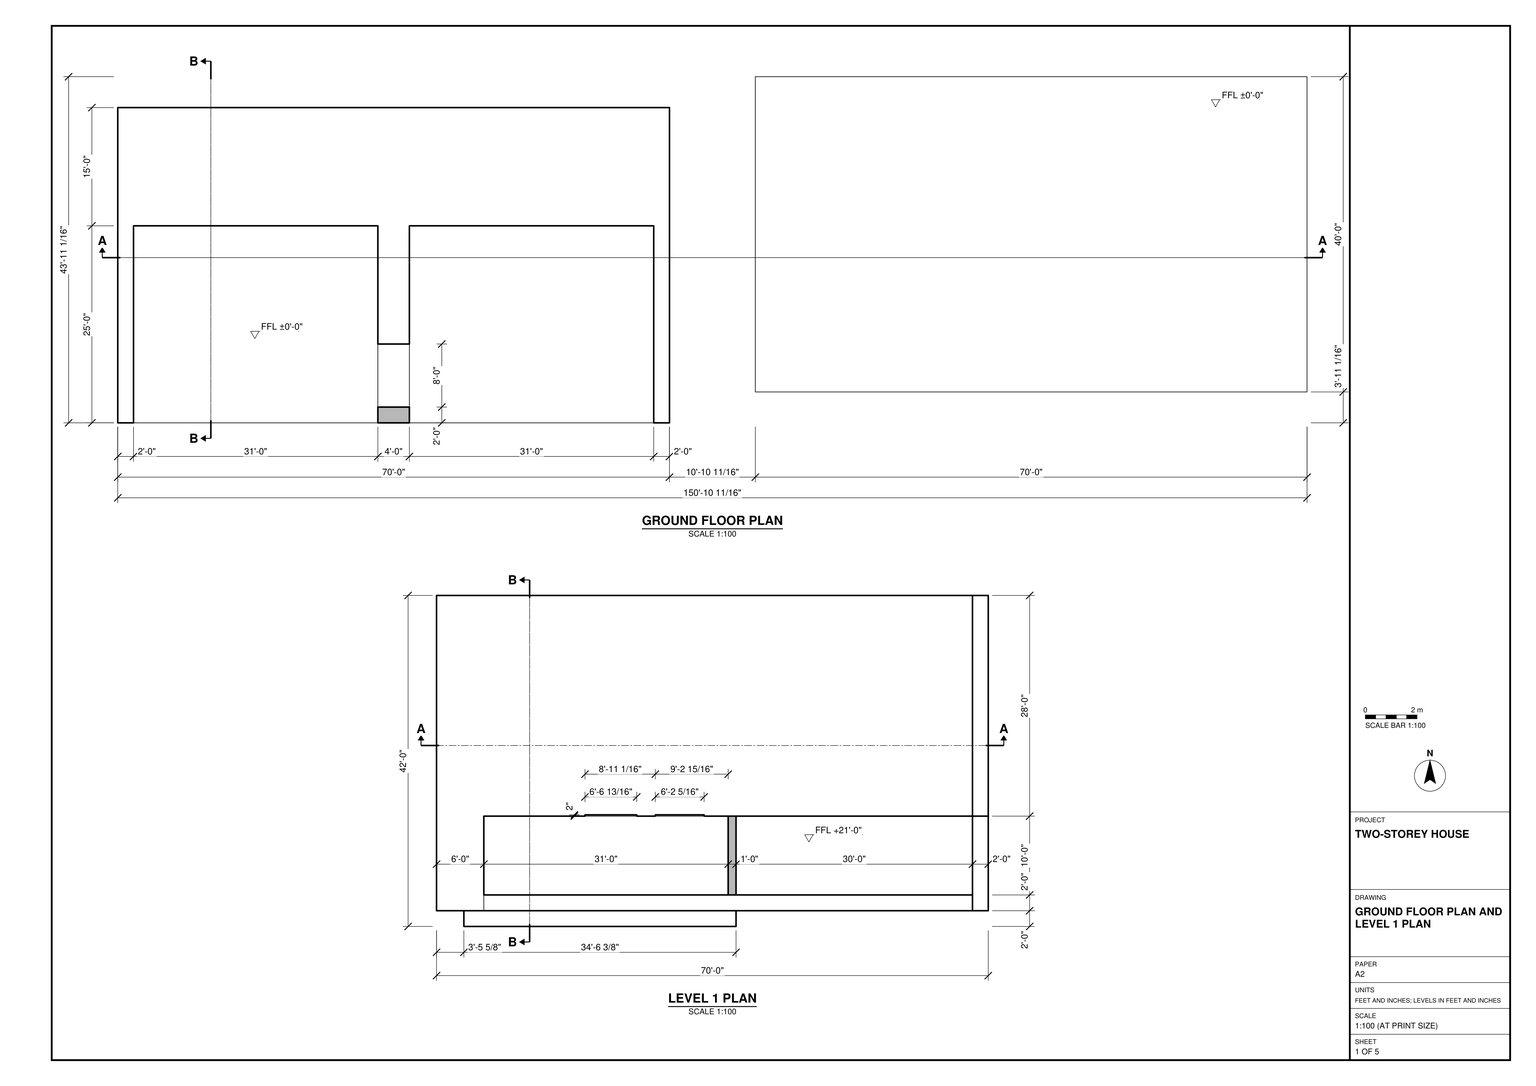
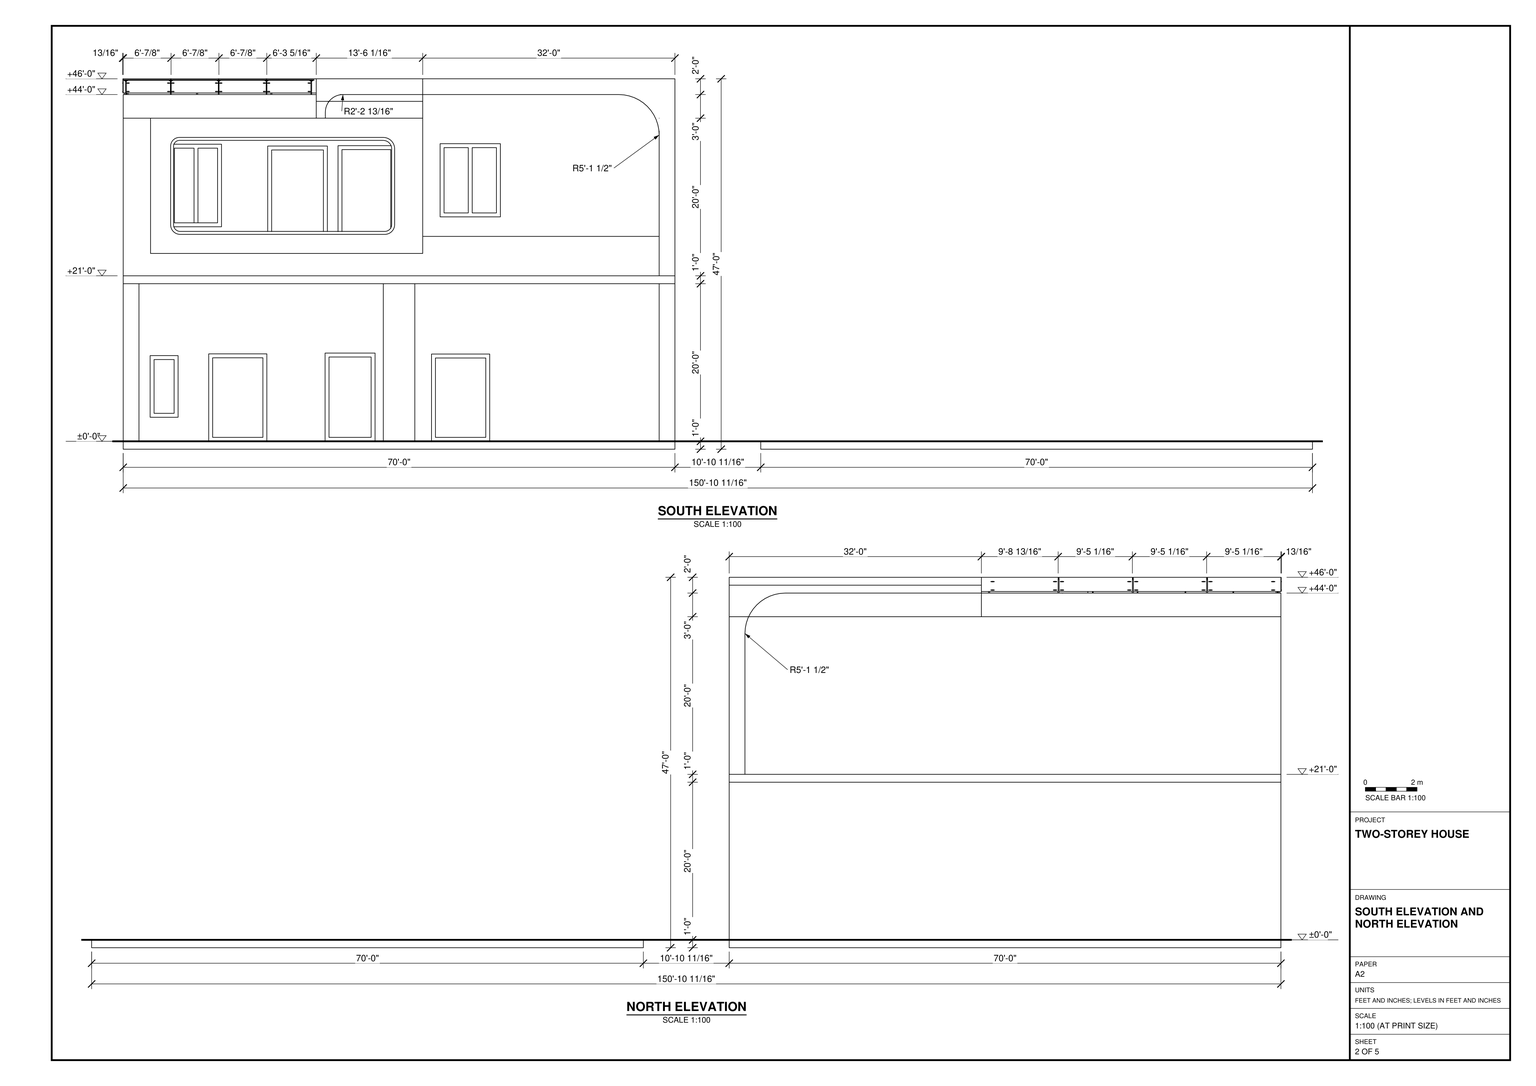
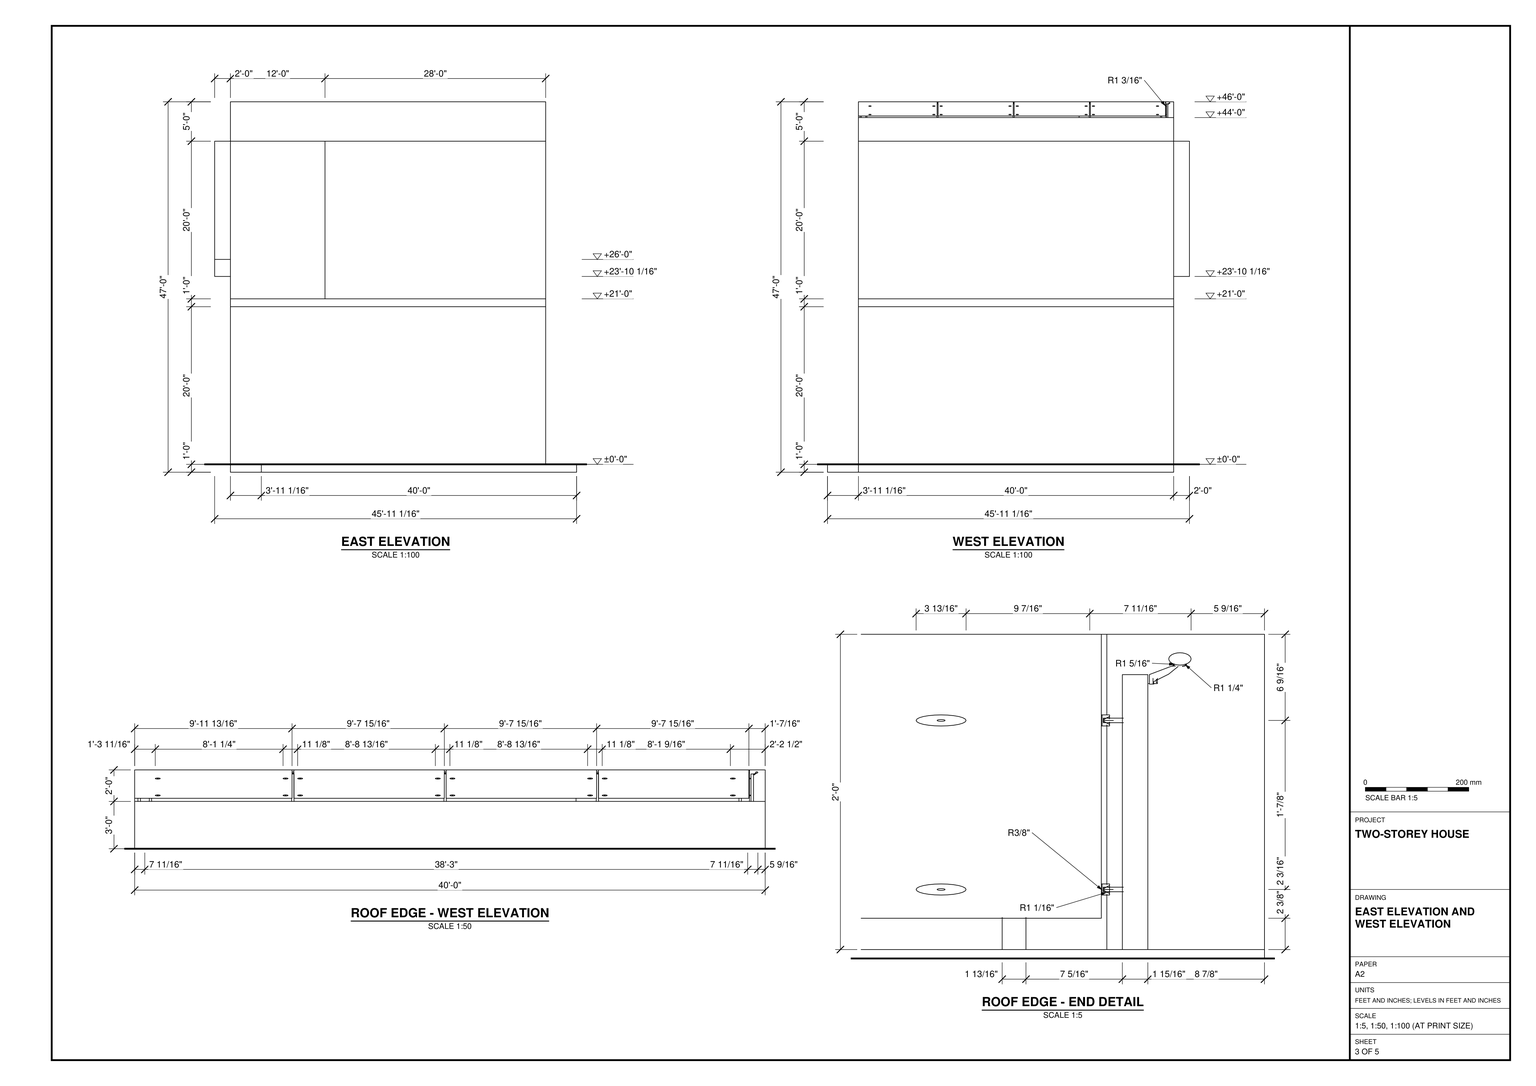
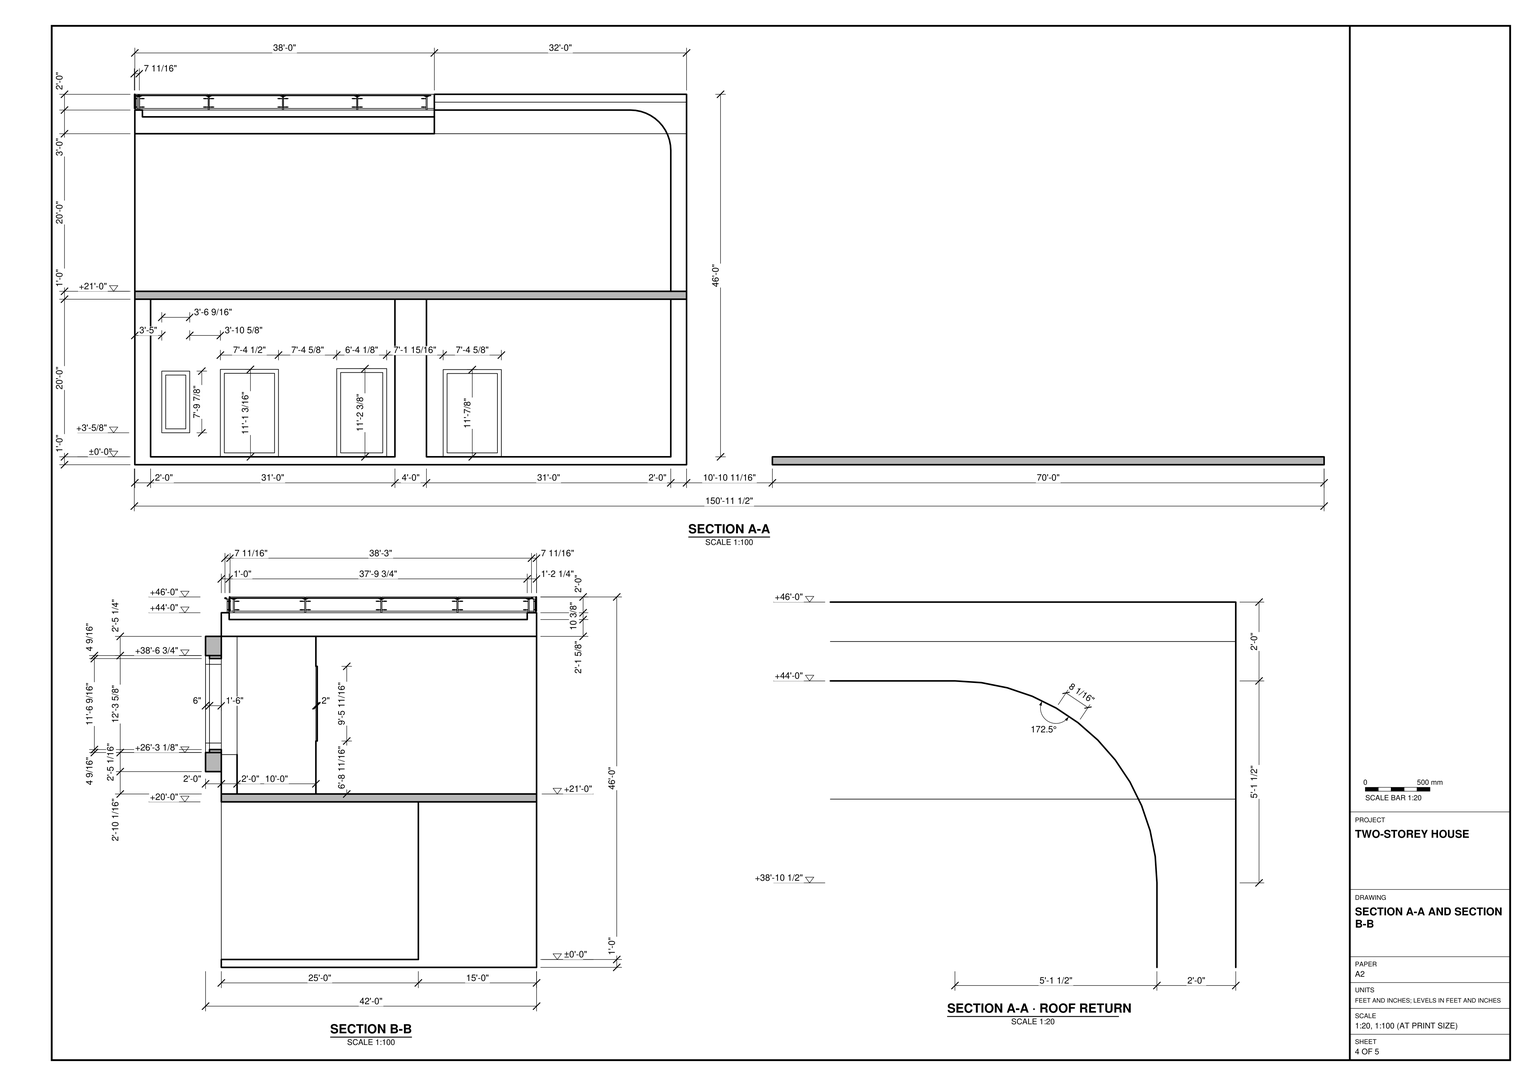
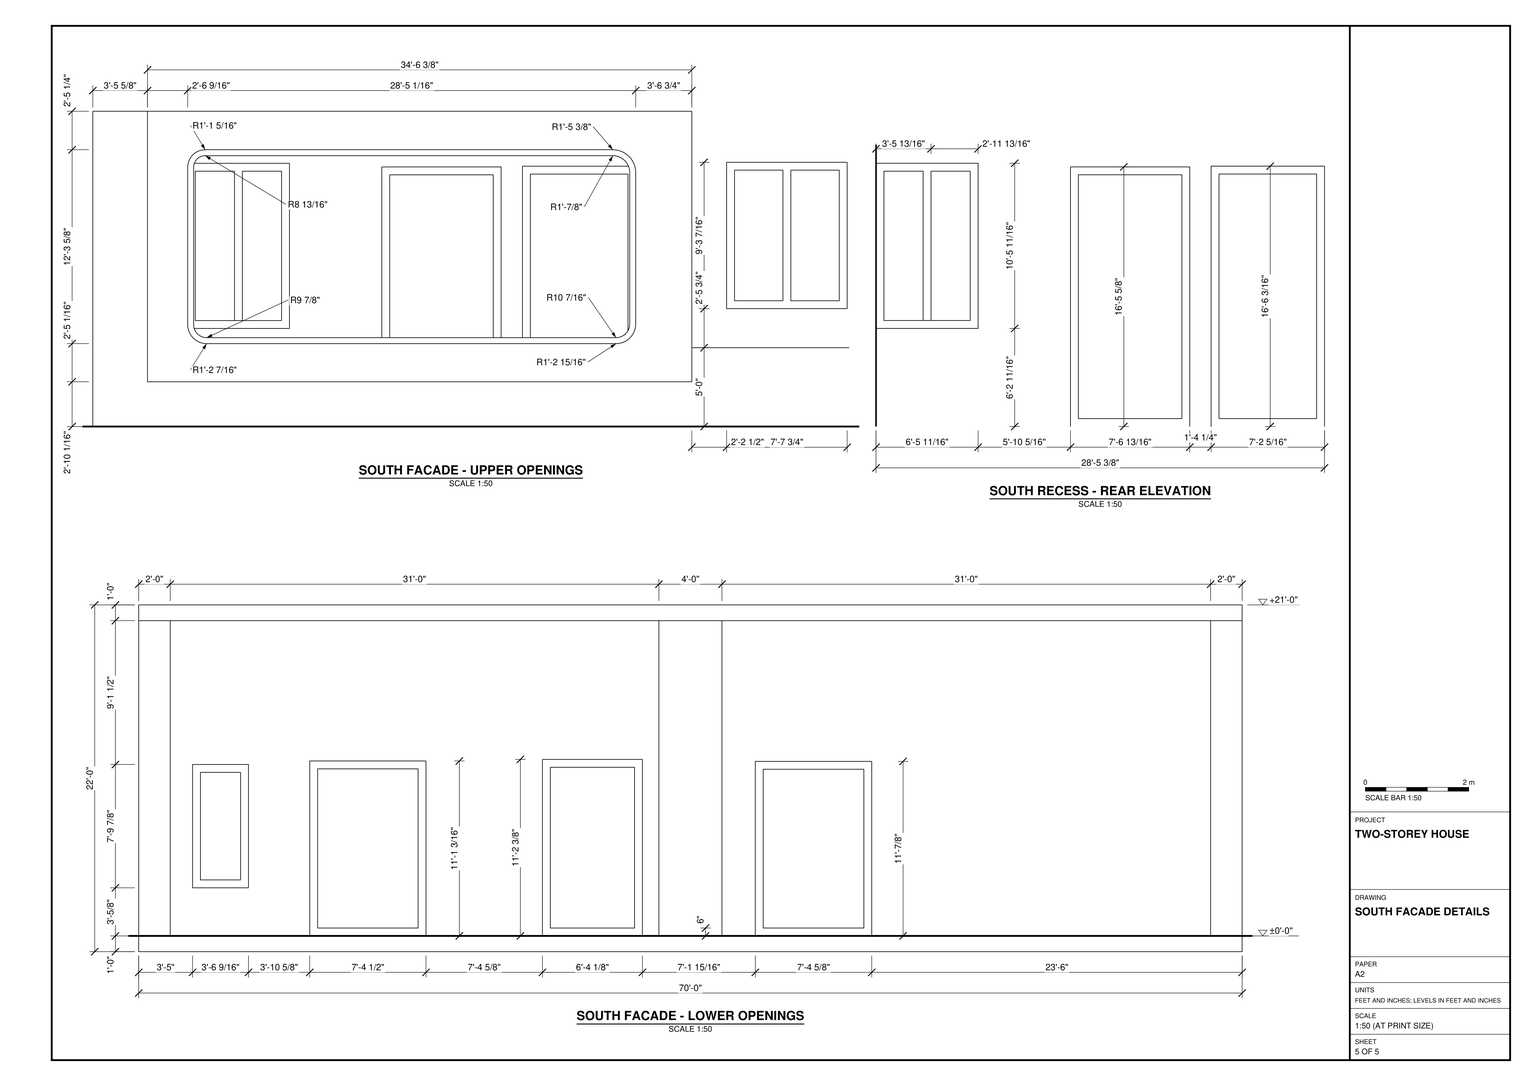
Build the two-storey house and the separate rectangular ground slab shown in task_files/diagram_01.pdf. Work in feet and inches. The complete model, including the offset slab, measures 150'-11 1/2" along X, 45'-11 1/16" along Y and 47'-0" along Z. Set the ground finished floor at ±0'-0" and the upper finished floor at +21'-0".

Use the ground floor plan to place the slab east of the house, with the gap and the northward offset shown. Build the walls, supports, floor slabs and flat roof to the thicknesses drawn. Form the two recessed bays on the south side and place the framed door and window openings on the walls behind the supports. On the upper storey, model the projecting surround with its rounded rectangular opening, keeping it distinct from the openings behind it. Form the curved return where the roof meets the right side of the south elevation. Use the roof-edge detail to model the glass guard panels, their point fixings and the handrail above the solid roof-edge band.

Keep walls, slabs and roof elements in separate groups or components. Keep any furniture or joinery piece separate and use components for repeated parts such as guard fittings. Any decor or loose items shown may be suitable library components. Save one SketchUp model as output_files/two_storey_house_with_a_glazed_roof_edge_guard.skp.

# SketchUp Ruby script. Lengths in inches.
U = 1.inch
M = Sketchup.active_model
def pt(a) = Geom::Point3d.new(a.map { |v| v * U })
def face(e, loops, mat)
  f = e.add_face(loops[0].map { |a| pt(a) })
  loops[1..].each { |l| e.add_face(l.map { |a| pt(a) }).erase! }
  f.material = f.back_material = mat if mat
  f
end
# faces: each face lists its corners as indices into pts; further lists are holes
def faces(e, pts, list, mat = nil) = list.each { |f| face(e, (f[0].is_a?(Array) ? f : [f]).map { |l| l.map { |i| pts[i] } }, mat) }
# xy, xz, yz: faces in a plane at the given z, y or x. An outline is a flat list of corners, or four numbers for a rectangle; further outlines are holes
def ring(l) = l.size == 4 ? [[l[0], l[1]], [l[2], l[1]], [l[2], l[3]], [l[0], l[3]]] : l.each_slice(2).to_a
def flat(e, list, mat, &to3) = list.each { |f| face(e, (f[0].is_a?(Array) ? f : [f]).map { |l| ring(l).map { |u, v| to3.(u, v) } }, mat) }
def xy(e, z, list, mat = nil) = flat(e, list, mat) { |x, y| [x, y, z] }
def xz(e, y, list, mat = nil) = flat(e, list, mat) { |x, z| [x, y, z] }
def yz(e, x, list, mat = nil) = flat(e, list, mat) { |y, z| [x, y, z] }
def lines(e, pts, list) = list.each { |a, b| e.add_line(pt(pts[a]), pt(pts[b])) }
# prism: a flat outline (further loops are holes) pulled along v
def prism(e, loops, v, mat = nil)
  f = face(e, loops, mat); d = Geom::Vector3d.new(v.map { |x| x * U })
  f.pushpull(f.normal.samedirection?(d) ? d.length : -d.length)
end
def box(e, o, s, mat = nil) = prism(e, [[o, [o[0] + s[0], o[1], o[2]], [o[0] + s[0], o[1] + s[1], o[2]], [o[0], o[1] + s[1], o[2]]]], [0, 0, s[2]], mat)
def at(x, y, z, deg = 0) = Geom::Transformation.translation(pt([x, y, z])) * Geom::Transformation.rotation(ORIGIN, Z_AXIS, deg.degrees)
def axes(o, x, y, z) = Geom::Transformation.new([*x, 0, *y, 0, *z, 0, *pt(o).to_a, 1])
def part(name) = M.definitions.add(name)
# library, detail: a bought-in or finely detailed component or shape, given as its bounding box
def library(name, o, s) = part(name).tap { |d| box(d.entities, o, s) }
def detail(e, o, s) = box(e.add_group.entities, o, s)
def put(e, d, t, mat = nil) = e.add_instance(d, t).tap { |i| i.material = mat if mat }
def group(e, t, mat = nil) = e.add_group.tap { |g| g.transformation = t; g.material = mat if mat }.entities
root = M.entities
M.materials.add("Translucent_Glass_Blue").color = [72, 237, 225]
M.materials["Translucent_Glass_Blue"].alpha = 0.08
M.materials.add("[0033_NavajoWhite]").color = [255, 222, 173]
M.materials.add("[0050_LemonChiffon]").color = [209, 205, 168]
M.materials.add("[Cladding Siding Tan]").color = [141, 143, 162]
M.materials.add("[Color I01]").color = [147, 170, 198]
M.materials.add("[Color I01]1").color = [97, 111, 135]
M.materials.add("[Color I08]").color = [0, 0, 102]
M.materials.add("[Color J01]").color = [174, 200, 234]
M.materials.add("[Color_002]").color = [198, 198, 198]
M.materials.add("[Color_007]").color = [89, 89, 89]
M.materials.add("[Wood_Cherry_Original]").color = [181, 109, 60]
c1 = library("componance C-15 handrail bracket",[0,0,0],[4.12,3.04,2.87])
c2 = library("C-13 Full Assembly",[0,0,0],[6.77,4.22,1.58])
c3 = part("C-13 Gasket")
prism(c3.entities,[[[0.79,0.0625,1.57],[0.99,0.0625,1.55],[1.18,0.0625,1.47],[1.34,0.0625,1.34],[1.47,0.0625,1.18],[1.55,0.0625,0.99],[1.57,0.0625,0.79],[1.55,0.0625,0.58],[1.47,0.0625,0.39],[1.34,0.0625,0.23],[1.18,0.0625,0.11],[0.99,0.0625,0.03],[0.79,0.0625,0],[0.58,0.0625,0.03],[0.39,0.0625,0.11],[0.23,0.0625,0.23],[0.11,0.0625,0.39],[0.03,0.0625,0.58],[0,0.0625,0.79],[0.03,0.0625,0.99],[0.11,0.0625,1.18],[0.23,0.0625,1.34],[0.39,0.0625,1.47],[0.58,0.0625,1.55]],[[0.91,0.0625,0.75],[0.91,0.0625,0.79],[0.91,0.0625,0.82],[0.9,0.0625,0.85],[0.875,0.0625,0.875],[0.85,0.0625,0.9],[0.82,0.0625,0.91],[0.79,0.0625,0.91],[0.75,0.0625,0.91],[0.72,0.0625,0.9],[0.7,0.0625,0.875],[0.68,0.0625,0.85],[0.67,0.0625,0.82],[0.66,0.0625,0.79],[0.67,0.0625,0.75],[0.68,0.0625,0.72],[0.7,0.0625,0.7],[0.72,0.0625,0.68],[0.75,0.0625,0.67],[0.79,0.0625,0.66],[0.82,0.0625,0.67],[0.85,0.0625,0.68],[0.875,0.0625,0.7],[0.9,0.0625,0.72]]],[0,-0.0625,0],"[Color_007]")
c4 = library("C-13 C",[0,0,0],[3.01,3.25,1.57])
c5 = library("componance half c-13",[0,0,0],[3.01,4.22,1.57])
c6 = part("C-13 Button")
prism(c6.entities,[[[0.79,0.34,1.57],[0.99,0.34,1.55],[1.18,0.34,1.47],[1.34,0.34,1.34],[1.47,0.34,1.18],[1.55,0.34,0.99],[1.57,0.34,0.79],[1.55,0.34,0.58],[1.47,0.34,0.39],[1.34,0.34,0.23],[1.18,0.34,0.11],[0.99,0.34,0.03],[0.79,0.34,0],[0.58,0.34,0.03],[0.39,0.34,0.11],[0.23,0.34,0.23],[0.11,0.34,0.39],[0.03,0.34,0.58],[0,0.34,0.79],[0.03,0.34,0.99],[0.11,0.34,1.18],[0.23,0.34,1.34],[0.39,0.34,1.47],[0.58,0.34,1.55]],[[0.91,0.34,0.79],[0.91,0.34,0.82],[0.9,0.34,0.85],[0.875,0.34,0.875],[0.85,0.34,0.9],[0.82,0.34,0.91],[0.79,0.34,0.91],[0.75,0.34,0.91],[0.72,0.34,0.9],[0.7,0.34,0.875],[0.68,0.34,0.85],[0.67,0.34,0.82],[0.66,0.34,0.79],[0.67,0.34,0.75],[0.68,0.34,0.72],[0.7,0.34,0.7],[0.72,0.34,0.68],[0.75,0.34,0.67],[0.79,0.34,0.66],[0.82,0.34,0.67],[0.85,0.34,0.68],[0.875,0.34,0.7],[0.9,0.34,0.72],[0.91,0.34,0.75]]],[0,-0.34,0],"[Color_002]")
c7 = part("Group\#3")
box(c7.entities,[65.66,0.29,4.71],[64.85,0.35,42.74],"Translucent_Glass_Blue")
prism(c7.entities,[[[261.82,4.8125,42.85],[261.82,4.97,42.82],[261.82,5.13,42.85],[261.82,5.28,42.94],[261.82,5.41,43.09],[261.82,5.51,43.28],[261.82,5.57,43.51],[261.82,5.59,43.75],[261.82,5.57,43.99],[261.82,5.51,44.21],[261.82,5.41,44.4],[261.82,5.28,44.55],[261.82,5.13,44.64],[261.82,4.97,44.67],[261.82,4.8125,44.64],[261.82,4.67,44.55],[261.82,4.54,44.4],[261.82,4.44,44.21],[261.82,4.38,43.99],[261.82,4.36,43.75],[261.82,4.38,43.51],[261.82,4.44,43.28],[261.82,4.54,43.09],[261.82,4.67,42.94]]],[-261.82,0,0],"[Wood_Cherry_Original]")
box(c7.entities,[131.31,0.29,4.71],[64.86,0.35,42.74],"Translucent_Glass_Blue")
box(c7.entities,[0,0.29,4.71],[64.86,0.35,42.74],"Translucent_Glass_Blue")
box(c7.entities,[196.97,0.29,4.71],[67.85,0.35,42.74],"Translucent_Glass_Blue")
xy(c7.entities,41.38,[[3.25,1.8,4.27,3.2],[64.8,1.8,65.83,3.2],[130.46,1.8,131.48,3.2],[196.11,1.8,197.14,3.2],[257.49,1.8,258.52,3.2]])
xz(c7.entities,1.8,[[3.25,0,4.27,41.38],[64.8,0,65.83,41.38],[130.46,0,131.48,41.38],[196.11,0,197.14,41.38],[257.49,0,258.52,41.38]])
xz(c7.entities,3.2,[[3.25,0,4.27,41.38],[64.8,0,65.83,41.38],[130.46,0,131.48,41.38],[196.11,0,197.14,41.38],[257.49,0,258.52,41.38]])
yz(c7.entities,3.25,[[1.8,0,3.2,41.38]])
yz(c7.entities,4.27,[[1.8,0,3.2,41.38]])
yz(c7.entities,64.8,[[1.8,0,3.2,35.02],[1.8,35.02,3.2,41.38]])
yz(c7.entities,65.83,[[1.8,0,3.2,35.02],[1.8,35.02,3.2,41.38]])
yz(c7.entities,130.46,[[1.8,0,3.2,35.02],[1.8,35.02,3.2,41.38]])
yz(c7.entities,131.48,[[1.8,0,3.2,41.38]])
yz(c7.entities,196.11,[[1.8,0,3.2,35.02],[1.8,35.02,3.2,41.38]])
yz(c7.entities,197.14,[[1.8,0,3.2,35.02],[1.8,35.02,3.2,41.38]])
yz(c7.entities,257.49,[[1.8,0,3.2,41.38]])
yz(c7.entities,258.52,[[1.8,0,3.2,41.38]])
p = [[196.85,0.29,4.71],[196.85,0.64,4.71],[65.54,0.29,4.71],[65.54,0.64,4.71]]
lines(c7.entities,p,[[0,1],[2,3]])
put(c7.entities,c1,axes([260.83,5.34,39.95],[-1.36782,0,0],[0,-0.7031,0],[0,0,1.06018]))
put(c7.entities,c2,axes([60.68,0,33.65],[1.36782,0,0],[0,0.7031,0],[0,0,1.06018]))
put(c7.entities,c2,axes([192,0,33.65],[1.36782,0,0],[0,0.7031,0],[0,0,1.06018]))
put(c7.entities,c1,axes([133.79,5.34,39.95],[-1.36782,0,0],[0,-0.7031,0],[0,0,1.06018]))
put(c7.entities,c1,axes([6.58,5.34,39.95],[-1.36782,0,0],[0,-0.7031,0],[0,0,1.06018]))
put(c7.entities,c3,axes([253.78,0.24,33.66],[1.36782,0,0],[0,0.7031,0],[0,0,1.06018]))
put(c7.entities,c2,axes([60.68,0,8.21],[1.36782,0,0],[0,0.7031,0],[0,0,1.06018]))
put(c7.entities,c4,axes([253.375,0.68,8.21],[1.36782,0,0],[0,0.7031,0],[0,0,1.06018]))
put(c7.entities,c5,axes([4.27,0,33.65],[1.36782,0,0],[0,0.7031,0],[0,0,1.06018]))
put(c7.entities,c6,axes([253.78,0,33.66],[1.36782,0,0],[0,0.7031,0],[0,0,1.06018]))
put(c7.entities,c3,axes([253.78,0.64,33.66],[1.36782,0,0],[0,0.7031,0],[0,0,1.06018]))
put(c7.entities,c2,axes([192,0,8.21],[1.36782,0,0],[0,0.7031,0],[0,0,1.06018]))
put(c7.entities,c2,axes([126.34,0,33.65],[1.36782,0,0],[0,0.7031,0],[0,0,1.06018]))
put(c7.entities,c2,axes([126.34,0,8.21],[1.36782,0,0],[0,0.7031,0],[0,0,1.06018]))
put(c7.entities,c5,axes([4.27,0,8.21],[1.36782,0,0],[0,0.7031,0],[0,0,1.06018]))
put(c7.entities,c6,axes([253.78,0,8.21],[1.36782,0,0],[0,0.7031,0],[0,0,1.06018]))
put(c7.entities,c3,axes([253.78,0.24,8.21],[1.36782,0,0],[0,0.7031,0],[0,0,1.06018]))
put(c7.entities,c4,axes([253.375,0.68,33.66],[1.36782,0,0],[0,0.7031,0],[0,0,1.06018]))
put(c7.entities,c1,axes([199.45,5.34,39.95],[-1.36782,0,0],[0,-0.7031,0],[0,0,1.06018]))
put(c7.entities,c3,axes([253.78,0.64,8.21],[1.36782,0,0],[0,0.7031,0],[0,0,1.06018]))
put(c7.entities,c1,axes([68.14,5.34,39.95],[-1.36782,0,0],[0,-0.7031,0],[0,0,1.06018]))
xy(root,0,[[0.82,24,840.82,504]])
xy(root,12,[[396.82,24,444.82,48],[396.82,48,444.82,144]])
xy(root,12,[[24.82,24,396.82,324],[444.82,24,816.82,324]],"[0033_NavajoWhite]")
xy(root,252,[[0.82,24,0.82,504,840.82,504,840.82,24,816.82,24,816.82,324,24.82,324,24.82,24],[396.82,24,444.82,48],[396.82,144,444.82,324],[396.82,144,444.82,324]])
xy(root,252,[[24.82,24,24.82,324,396.82,324,396.82,144,444.82,144,444.82,324,816.82,324,816.82,24,444.82,24,444.82,48,396.82,48,396.82,24]],"[0033_NavajoWhite]")
xy(root,264,[[0.82,24,0.82,504,840.82,504,840.82,168,72.82,168,72.82,24],[72.82,24,816.82,48],[816.82,24,840.82,168],[456.82,48,816.82,168]])
xy(root,264,[[72.82,48,444.82,168]],"[0033_NavajoWhite]")
xy(root,264.01,[[816.82,24,840.82,168],[816.82,168,840.82,504]])
xy(root,270,[[226.82,168,305.63,170],[333.89,168,408.2,170]])
xy(root,298.0625,[[42.44,0,456.82,24]])
xy(root,324,[[456.82,24,816.82,48]],"[Color J01]")
xy(root,327.11,[[87.47,6,399.125,24]])
xy(root,327.11,[[87.47,0,399.125,6]],"[Color I01]")
xy(root,331.65,[[87.47,6,399.125,24]],"[0033_NavajoWhite]")
xy(root,344.67,[[114.66,168,144.5,170]])
xy(root,359.74,[[489.31,168,526.18,170],[532.18,168,569.06,170]])
xy(root,455.625,[[226.82,168,305.63,170]])
xy(root,456.1875,[[333.89,168,408.2,170]])
xy(root,458.37,[[114.66,168,144.5,170]])
xy(root,459.18,[[489.31,168,526.18,170],[532.18,168,569.06,170]])
xy(root,470.19,[[86.36,6,396.6875,24]],"[0033_NavajoWhite]")
xy(root,474.73,[[86.36,6,396.6875,24]])
xy(root,474.73,[[86.36,0,396.6875,6]],"[Color I01]")
xy(root,504,[[42.44,0,72.82,24],[72.82,0,444.82,24],[444.82,0,456.82,24],[444.82,24,456.82,48],[444.82,48,456.82,168]])
xy(root,504,[[0.82,24,0.82,504,456.82,504,456.82,168,72.82,168,72.82,24],[72.82,24,444.82,168]],"[0033_NavajoWhite]")
xy(root,529.625,[[314.21,24,456.82,24,456.82,489.75,12.38,489.75,12.38,36,314.21,36],[294.75,24,313.1,36],[313.1,24,314.21,36]])
xy(root,540.01,[[0.82,24,294.75,24,294.75,36,12.38,36,12.38,489.75,456.82,489.75,456.82,504,0.82,504],[335.39,24,456.82,36]])
xy(root,540.01,[[456.82,24,755.31,504]],"[Color J01]")
xy(root,564.01,[[294.75,24,456.82,36],[456.82,24,840.82,504]])
xz(root,0,[[[42.44,298.0625,456.82,504],[87.47,327.11,85.59,327.23,83.73,327.6,81.94,328.21,80.25,329.05,78.68,330.09,77.26,331.34,76.01,332.76,74.96,334.33,74.125,336.03,73.52,337.82,73.15,339.67,73.03,341.55,73.03,461.4,73.14,463.14,73.48,464.85,74.04,466.5,74.8125,468.07,75.78,469.52,76.93,470.83,78.24,471.98,79.69,472.95,81.26,473.72,82.91,474.28,84.62,474.62,86.36,474.73,396.6875,474.73,398.96,474.59,401.19,474.14,403.35,473.41,405.39,472.4,407.28,471.14,408.99,469.64,410.49,467.93,411.76,466.03,412.76,463.99,413.5,461.84,413.94,459.6,414.09,457.33,414.09,342.07,413.96,340.12,413.58,338.2,412.95,336.35,412.08,334.59,411,332.96,409.71,331.49,408.23,330.2,406.61,329.11,404.85,328.25,403,327.62,401.08,327.24,399.125,327.11]]],"[Color I01]")
xz(root,6,[[[87.47,327.11,399.125,327.11,401.08,327.24,403,327.62,404.85,328.25,406.61,329.11,408.23,330.2,409.71,331.49,411,332.96,412.08,334.59,412.95,336.35,413.58,338.2,413.96,340.12,414.09,342.07,414.09,457.33,413.94,459.6,413.5,461.84,412.76,463.99,411.76,466.03,410.49,467.93,408.99,469.64,407.28,471.14,405.39,472.4,403.35,473.41,401.19,474.14,398.96,474.59,396.6875,474.73,86.36,474.73,84.62,474.62,82.91,474.28,81.26,473.72,79.69,472.95,78.24,471.98,76.93,470.83,75.78,469.52,74.8125,468.07,74.04,466.5,73.48,464.85,73.14,463.14,73.03,461.4,73.03,341.55,73.15,339.67,73.52,337.82,74.125,336.03,74.96,334.33,76.01,332.76,77.26,331.34,78.68,330.09,80.25,329.05,81.94,328.21,83.73,327.6,85.59,327.23],[87.47,331.65,86.18,331.73,84.91,331.99,83.68,332.4,82.52,332.98,81.44,333.7,80.47,334.55,79.61,335.53,78.89,336.6,78.32,337.76,77.9,338.99,77.65,340.26,77.57,341.55,77.57,461.4,77.64,462.55,77.87,463.68,78.24,464.77,78.75,465.8,79.38,466.75,80.14,467.62,81.01,468.38,81.96,469.02,83,469.52,84.09,469.89,85.21,470.12,86.36,470.19,396.6875,470.19,398.37,470.08,400.02,469.76,401.61,469.22,403.12,468.47,404.52,467.54,405.78,466.43,406.89,465.16,407.83,463.76,408.57,462.26,409.11,460.66,409.4375,459.01,409.55,457.33,409.55,342.07,409.46,340.71,409.19,339.375,408.76,338.09,408.15,336.86,407.39,335.73,406.5,334.7,405.47,333.8,404.34,333.05,403.11,332.44,401.82,332.01,400.49,331.74,399.125,331.65]]],"[0050_LemonChiffon]")
xz(root,24,[[0.82,252,840.82,264],[816.82,264,840.82,264.01],[[42.44,298.0625,456.82,504],[87.47,327.11,399.125,327.11,401.08,327.24,403,327.62,404.85,328.25,406.61,329.11,408.23,330.2,409.71,331.49,411,332.96,412.08,334.59,412.95,336.35,413.58,338.2,413.96,340.12,414.09,342.07,414.09,457.33,413.94,459.6,413.5,461.84,412.76,463.99,411.76,466.03,410.49,467.93,408.99,469.64,407.28,471.14,405.39,472.4,403.35,473.41,401.19,474.14,398.96,474.59,396.6875,474.73,86.36,474.73,84.62,474.62,82.91,474.28,81.26,473.72,79.69,472.95,78.24,471.98,76.93,470.83,75.78,469.52,74.8125,468.07,74.04,466.5,73.48,464.85,73.14,463.14,73.03,461.4,73.03,341.55,73.15,339.67,73.52,337.82,74.125,336.03,74.96,334.33,76.01,332.76,77.26,331.34,78.68,330.09,80.25,329.05,81.94,328.21,83.73,327.6,85.59,327.23]],[[87.47,327.11,85.59,327.23,83.73,327.6,81.94,328.21,80.25,329.05,78.68,330.09,77.26,331.34,76.01,332.76,74.96,334.33,74.125,336.03,73.52,337.82,73.15,339.67,73.03,341.55,73.03,461.4,73.14,463.14,73.48,464.85,74.04,466.5,74.8125,468.07,75.78,469.52,76.93,470.83,78.24,471.98,79.69,472.95,81.26,473.72,82.91,474.28,84.62,474.62,86.36,474.73,396.6875,474.73,398.96,474.59,401.19,474.14,403.35,473.41,405.39,472.4,407.28,471.14,408.99,469.64,410.49,467.93,411.76,466.03,412.76,463.99,413.5,461.84,413.94,459.6,414.09,457.33,414.09,342.07,413.96,340.12,413.58,338.2,412.95,336.35,412.08,334.59,411,332.96,409.71,331.49,408.23,330.2,406.61,329.11,404.85,328.25,403,327.62,401.08,327.24,399.125,327.11],[87.47,331.65,399.125,331.65,400.49,331.74,401.82,332.01,403.11,332.44,404.34,333.05,405.47,333.8,406.5,334.7,407.39,335.73,408.15,336.86,408.76,338.09,409.19,339.375,409.46,340.71,409.55,342.07,409.55,457.33,409.4375,459.01,409.11,460.66,408.57,462.26,407.83,463.76,406.89,465.16,405.78,466.43,404.52,467.54,403.12,468.47,401.61,469.22,400.02,469.76,398.37,470.08,396.6875,470.19,86.36,470.19,85.21,470.12,84.09,469.89,83,469.52,81.96,469.02,81.01,468.38,80.14,467.62,79.38,466.75,78.75,465.8,78.24,464.77,77.87,463.68,77.64,462.55,77.57,461.4,77.57,341.55,77.65,340.26,77.9,338.99,78.32,337.76,78.89,336.6,79.61,335.53,80.47,334.55,81.44,333.7,82.52,332.98,83.68,332.4,84.91,331.99,86.18,331.73]],[313.1,528,314.11,529.51,314.21,529.625,313.1,529.625]])
xz(root,24,[[0.82,0,840.82,0,840.82,252,816.82,252,816.82,12,24.82,12,24.82,252,0.82,252],[396.82,12,444.82,252]],"[Color I01]1")
xz(root,24,[[0.82,264,816.82,264,816.82,324,456.82,324,456.82,298.0625,42.44,298.0625,42.44,504,0.82,504],[816.82,264.01,840.82,264.01,840.82,564.01,456.82,564.01,456.82,540.01,755.31,540.01,763.34,539.48,771.23,537.91,778.85,535.33,786.0625,531.77,792.75,527.3,798.8,522,804.11,515.95,808.58,509.26,812.13,502.04,814.72,494.42,816.29,486.53,816.82,478.5],[0.82,504,294.75,540.01],[294.75,504,308.57,504,308.57,513.18,308.8,516.6875,309.48,520.13,310.61,523.45,312.16,526.6,313.1,528,313.1,529.625,294.75,529.625],[308.57,504,456.82,504,456.82,529.625,314.21,529.625,314.11,529.51,313.1,528,312.16,526.6,310.61,523.45,309.48,520.13,308.8,516.6875,308.57,513.18],
  [294.75,529.625,314.21,529.625,316.42,532.15,319.0625,534.47,321.98,536.42,325.125,537.97,328.45,539.1,331.89,539.78,335.39,540.01,456.82,540.01,456.82,564.01,294.75,564.01]],"[Color J01]")
xz(root,36,[[12.38,529.625,294.75,540.01],[294.75,529.625,294.75,564.01,456.82,564.01,456.82,540.01,335.39,540.01,331.89,539.78,328.45,539.1,325.125,537.97,321.98,536.42,319.0625,534.47,316.42,532.15,314.21,529.625]])
xz(root,48,[[396.82,12,444.82,252],[444.82,264,456.82,324],[456.82,264,816.82,324],[444.82,324,456.82,504]])
xz(root,48,[[72.82,264,444.82,324]],"[0033_NavajoWhite]")
xz(root,144,[[396.82,12,444.82,252]])
xz(root,168,[[444.82,264,456.82,504],[816.82,264,840.82,264.01],[816.82,264.01,840.82,504],[78.82,344.67,108.66,458.37]])
xz(root,168,[[72.82,264,220.82,264,220.82,461.625,311.63,461.625,311.63,264,327.89,264,327.89,462.1875,414.2,462.1875,414.2,264,444.82,264,444.82,504,72.82,504,72.82,464.37,150.5,464.37,150.5,338.67,72.82,338.67]],"[0033_NavajoWhite]")
xz(root,168,[[[456.82,264,816.82,552],[483.31,353.74,575.06,465.18]]],"[Cladding Siding Tan]")
xz(root,168,[[[220.82,264,311.63,461.625],[226.82,270,305.63,455.625]],[[327.89,264,414.2,462.1875],[333.89,270,408.2,456.1875]],[[72.82,338.67,150.5,464.37],[78.82,344.67,78.82,458.37,108.66,458.37,108.66,344.67,114.66,344.67,114.66,458.37,144.5,458.37,144.5,344.67]],[[483.31,353.74,575.06,465.18],[489.31,359.74,526.18,459.18],[532.18,359.74,569.06,459.18]]],"[Color I08]")
xz(root,170,[[226.82,270,305.63,455.625],[333.89,270,408.2,456.1875],[114.66,344.67,144.5,458.37],[489.31,359.74,526.18,459.18],[532.18,359.74,569.06,459.18]])
xz(root,324,[[137.02,18,213.52,139.1875],[314.17,18,378.29,140.375],[476.21,18,552.84,138.875],[47.8125,54.63,78.375,136.51]])
xz(root,324,[[[24.82,12,131.02,12,131.02,145.1875,219.52,145.1875,219.52,12,308.17,12,308.17,146.375,384.29,146.375,384.29,12,396.82,12,396.82,252,24.82,252],[41.8125,48.63,84.375,142.51]],[444.82,12,470.21,12,470.21,144.875,558.84,144.875,558.84,12,816.82,12,816.82,252,444.82,252]],"[0033_NavajoWhite]")
xz(root,324,[[[131.02,12,219.52,145.1875],[137.02,18,213.52,139.1875]],[[308.17,12,384.29,146.375],[314.17,18,378.29,140.375]],[[470.21,12,558.84,144.875],[476.21,18,552.84,138.875]],[[41.8125,48.63,84.375,142.51],[47.8125,54.63,78.375,136.51]]],"[Color I08]")
xz(root,489.75,[[12.38,529.625,456.82,540.01]])
xz(root,504,[[0.82,0,840.82,252],[0.82,252,840.82,264],[0.82,264,0.82,504,811.17,504,812.13,502.04,814.72,494.42,816.29,486.53,816.82,478.5,816.82,264.01,840.82,264.01,840.82,264],[816.82,264.01,816.82,478.5,816.29,486.53,814.72,494.42,812.13,502.04,811.17,504,840.82,504,840.82,264.01],[0.82,504,456.82,540.01],
  [456.82,504,456.82,540.01,755.31,540.01,763.34,539.48,771.23,537.91,778.85,535.33,786.0625,531.77,792.75,527.3,798.8,522,804.11,515.95,808.58,509.26,811.17,504],[811.17,504,808.58,509.26,804.11,515.95,798.8,522,792.75,527.3,786.0625,531.77,778.85,535.33,771.23,537.91,763.34,539.48,755.31,540.01,456.82,540.01,456.82,552,840.82,552,840.82,504],[456.82,552,840.82,564.01]])
yz(root,0.82,[[24,0,504,252],[24,252,504,264],[24,504,504,540.01]])
yz(root,0.82,[[24,264,504,504]],"[0033_NavajoWhite]")
yz(root,12.38,[[36,529.625,489.75,540.01]])
yz(root,24.82,[[24,12,324,252]],"[0033_NavajoWhite]")
yz(root,42.44,[[0,298.0625,24,504]])
yz(root,72.82,[[48,264,168,504]],"[0033_NavajoWhite]")
yz(root,73.03,[[6,341.55,24,461.4]])
yz(root,73.03,[[0,341.55,6,461.4]],"[Color I01]")
yz(root,77.57,[[6,341.55,24,461.4]],"[0033_NavajoWhite]")
yz(root,114.66,[[168,344.67,170,458.37]])
yz(root,144.5,[[168,344.67,170,458.37]])
yz(root,226.82,[[168,270,170,455.625]])
yz(root,294.75,[[24,529.625,36,540.01],[24,540.01,36,564.01]])
yz(root,305.63,[[168,270,170,455.625]])
yz(root,333.89,[[168,270,170,456.1875]])
yz(root,396.82,[[24,12,48,252],[144,12,324,252]])
yz(root,408.2,[[168,270,170,456.1875]])
yz(root,409.55,[[6,342.07,24,457.33]],"[0033_NavajoWhite]")
yz(root,414.09,[[6,342.07,24,457.33]])
yz(root,414.09,[[0,342.07,6,457.33]],"[Color I01]")
yz(root,444.82,[[24,12,48,252],[144,12,324,252]])
yz(root,444.82,[[48,264,168,504]],"[0033_NavajoWhite]")
yz(root,456.82,[[48,264,168,504],[0,298.0625,24,324],[0,324,24,504],[24,324,48,504],[24,504,168,529.625],
  [168,504,504,504,504,540.01,489.75,540.01,489.75,529.625,168,529.625],[168,529.625,489.75,540.01],[24,540.01,36,564.01],[36,540.01,36,564.01,504,564.01,504,552,168,552,168,540.01],[168,540.01,504,552]])
yz(root,489.31,[[168,359.74,170,459.18]])
yz(root,526.18,[[168,359.74,170,459.18]])
yz(root,532.18,[[168,359.74,170,459.18]])
yz(root,569.06,[[168,359.74,170,459.18]])
yz(root,816.82,[[24,264,48,264.01],[48,264,168,264.01],[24,264.01,48,324],[168,264.01,504,478.5]])
yz(root,816.82,[[24,12,324,252]],"[0033_NavajoWhite]")
yz(root,816.82,[[48,264.01,48,324,24,324,24,478.5,168,478.5,168,264.01]],"[Color J01]")
yz(root,840.82,[[24,0,504,252],[24,252,504,264],[24,264,168,264.01],[168,264,504,264.01],[24,264.01,168,504],
  [168,264.01,504,504],[168,504,504,504,504,564.01,24,564.01,24,504.01,168,504.01],[24,504,168,504.01]])
p = [[87.47,0,327.11],[87.47,6,327.11],[85.59,6,327.23],[85.59,0,327.23],[401.08,0,327.24],[401.08,6,327.24],
  [399.125,6,327.11],[399.125,0,327.11],[87.47,24,327.11],[85.59,24,327.23],[401.08,24,327.24],[399.125,24,327.11],
  [83.73,6,327.6],[83.73,0,327.6],[403,0,327.62],[403,6,327.62],[83.73,24,327.6],[403,24,327.62],
  [81.94,6,328.21],[81.94,0,328.21],[404.85,0,328.25],[404.85,6,328.25],[81.94,24,328.21],[404.85,24,328.25],
  [80.25,6,329.05],[80.25,0,329.05],[406.61,0,329.11],[406.61,6,329.11],[80.25,24,329.05],[406.61,24,329.11],
  [78.68,6,330.09],[78.68,0,330.09],[78.68,24,330.09],[408.23,0,330.2],[408.23,6,330.2],[408.23,24,330.2],
  [77.26,6,331.34],[77.26,0,331.34],[77.26,24,331.34],[409.71,0,331.49],[409.71,6,331.49],[409.71,24,331.49],
  [76.01,6,332.76],[76.01,0,332.76],[76.01,24,332.76],[411,0,332.96],[411,6,332.96],[411,24,332.96],
  [86.18,24,331.73],[84.91,24,331.99],[84.91,6,331.99],[86.18,6,331.73],[87.47,24,331.65],[87.47,6,331.65],
  [400.49,24,331.74],[399.125,24,331.65],[399.125,6,331.65],[400.49,6,331.74],[401.82,24,332.01],[401.82,6,332.01],
  [83.68,24,332.4],[83.68,6,332.4],[403.11,24,332.44],[403.11,6,332.44],[82.52,24,332.98],[82.52,6,332.98],
  [404.34,24,333.05],[404.34,6,333.05],[74.96,6,334.33],[74.96,0,334.33],[74.96,24,334.33],[412.08,0,334.59],
  [412.08,6,334.59],[81.44,24,333.7],[81.44,6,333.7],[405.47,24,333.8],[405.47,6,333.8],[412.08,24,334.59],
  [80.47,24,334.55],[80.47,6,334.55],[406.5,24,334.7],[406.5,6,334.7],[74.125,6,336.03],[74.125,0,336.03],
  [74.125,24,336.03],[412.95,0,336.35],[412.95,6,336.35],[79.61,24,335.53],[79.61,6,335.53],[412.95,24,336.35],
  [407.39,24,335.73],[407.39,6,335.73],[78.89,24,336.6],[78.89,6,336.6],[408.15,24,336.86],[408.15,6,336.86],
  [73.52,6,337.82],[73.52,0,337.82],[73.52,24,337.82],[413.58,0,338.2],[413.58,6,338.2],[413.58,24,338.2],
  [78.32,24,337.76],[78.32,6,337.76],[408.76,24,338.09],[408.76,6,338.09],[73.15,6,339.67],[73.15,0,339.67],
  [73.15,24,339.67],[77.9,24,338.99],[77.9,6,338.99],[409.19,24,339.375],[409.19,6,339.375],[413.96,0,340.12],
  [413.96,6,340.12],[413.96,24,340.12],[77.65,24,340.26],[77.65,6,340.26],[409.46,24,340.71],[409.46,6,340.71],
  [73.03,6,341.55],[73.03,0,341.55],[73.03,24,341.55],[414.09,0,342.07],[414.09,6,342.07],[414.09,24,342.07],
  [77.57,24,341.55],[77.57,6,341.55],[409.55,24,342.07],[409.55,6,342.07],[413.94,0,459.6],[413.94,6,459.6],
  [414.09,6,457.33],[414.09,0,457.33],[409.4375,24,459.01],[409.55,24,457.33],[409.55,6,457.33],[409.4375,6,459.01],
  [413.94,24,459.6],[414.09,24,457.33],[409.11,24,460.66],[409.11,6,460.66],[413.5,0,461.84],[413.5,6,461.84],
  [413.5,24,461.84],[408.57,24,462.26],[408.57,6,462.26],[73.03,0,461.4],[73.03,6,461.4],[73.14,6,463.14],
  [73.14,0,463.14],[73.03,24,461.4],[73.14,24,463.14],[77.57,24,461.4],[77.64,24,462.55],[77.64,6,462.55],
  [77.57,6,461.4],[412.76,0,463.99],[412.76,6,463.99],[412.76,24,463.99],[407.83,24,463.76],[407.83,6,463.76],
  [77.87,24,463.68],[77.87,6,463.68],[73.48,6,464.85],[73.48,0,464.85],[73.48,24,464.85],[78.24,24,464.77],
  [78.24,6,464.77],[406.89,24,465.16],[406.89,6,465.16],[411.76,0,466.03],[411.76,6,466.03],[411.76,24,466.03],
  [78.75,24,465.8],[78.75,6,465.8],[74.04,6,466.5],[74.04,0,466.5],[74.04,24,466.5],[405.78,24,466.43],
  [405.78,6,466.43],[79.38,24,466.75],[79.38,6,466.75],[410.49,0,467.93],[410.49,6,467.93],[410.49,24,467.93],
  [404.52,24,467.54],[404.52,6,467.54],[74.8125,6,468.07],[74.8125,0,468.07],[74.8125,24,468.07],[80.14,24,467.62],
  [80.14,6,467.62],[403.12,24,468.47],[403.12,6,468.47],[81.01,24,468.38],[81.01,6,468.38],[408.99,0,469.64],
  [408.99,6,469.64],[408.99,24,469.64],[75.78,6,469.52],[75.78,0,469.52],[75.78,24,469.52],[81.96,24,469.02],
  [81.96,6,469.02],[401.61,24,469.22],[401.61,6,469.22],[83,24,469.52],[83,6,469.52],[400.02,24,469.76],
  [400.02,6,469.76],[76.93,6,470.83],[76.93,0,470.83],[76.93,24,470.83],[84.09,24,469.89],[84.09,6,469.89],
  [407.28,0,471.14],[407.28,6,471.14],[407.28,24,471.14],[398.37,24,470.08],[398.37,6,470.08],[85.21,24,470.12],
  [85.21,6,470.12],[86.36,24,470.19],[86.36,6,470.19],[396.6875,24,470.19],[396.6875,6,470.19],[78.24,6,471.98],
  [78.24,0,471.98],[78.24,24,471.98],[405.39,0,472.4],[405.39,6,472.4],[405.39,24,472.4],[79.69,6,472.95],
  [79.69,0,472.95],[79.69,24,472.95],[403.35,0,473.41],[403.35,6,473.41],[403.35,24,473.41],[81.26,6,473.72],
  [81.26,0,473.72],[81.26,24,473.72],[401.19,0,474.14],[401.19,6,474.14],[401.19,24,474.14],[82.91,6,474.28],
  [82.91,0,474.28],[82.91,24,474.28],[398.96,0,474.59],[398.96,6,474.59],[398.96,24,474.59],[84.62,6,474.62],
  [84.62,0,474.62],[84.62,24,474.62],[86.36,6,474.73],[86.36,0,474.73],[396.6875,0,474.73],[396.6875,6,474.73],
  [86.36,24,474.73],[396.6875,24,474.73],[816.82,24,478.5],[816.29,24,486.53],[816.29,504,486.53],[816.82,504,478.5],
  [816.82,168,478.5],[814.72,24,494.42],[814.72,504,494.42],[812.13,24,502.04],[812.13,504,502.04],[808.58,24,509.26],
  [808.58,504,509.26],[811.17,504,504],[804.11,24,515.95],[804.11,504,515.95],[798.8,24,522],[798.8,504,522],
  [792.75,24,527.3],[792.75,504,527.3],[786.0625,24,531.77],[786.0625,504,531.77],[316.42,24,532.15],[314.21,24,529.625],
  [314.21,36,529.625],[316.42,36,532.15],[778.85,24,535.33],[778.85,504,535.33],[319.0625,24,534.47],[319.0625,36,534.47],
  [321.98,24,536.42],[321.98,36,536.42],[771.23,24,537.91],[771.23,504,537.91],[325.125,24,537.97],[325.125,36,537.97],
  [763.34,24,539.48],[763.34,504,539.48],[328.45,24,539.1],[328.45,36,539.1],[331.89,24,539.78],[331.89,36,539.78],
  [755.31,24,540.01],[755.31,504,540.01],[335.39,24,540.01],[335.39,36,540.01],[816.82,48,504],[816.82,48,504.01],
  [816.82,24,504],[816.82,24,504.01],[816.82,168,552],[840.82,168,552],[72.82,48,324],[72.82,24,324],
  [444.82,48,324],[444.82,24,324],[456.82,24,529.625],[456.82,24,540.01]]
faces(root,p,[[0,1,2,3],[4,5,6,7],[3,2,12,13],[14,15,5,4],[13,12,18,19],[20,21,15,14],[19,18,24,25],[26,27,21,20],
  [25,24,30,31],[33,34,27,26],[31,30,36,37],[39,40,34,33],[37,36,42,43],[45,46,40,39],[43,42,68,69],[71,72,46,45],
  [69,68,82,83],[85,86,72,71],[83,82,96,97],[99,100,86,85],[97,96,106,107],[113,114,100,99],[107,106,120,121],[123,124,114,113],
  [130,131,132,133],[142,143,131,130],[147,148,149,150],[157,158,143,142],[150,149,164,165],[171,172,158,157],[165,164,176,177],[183,184,172,171],
  [177,176,188,189],[197,198,184,183],[189,188,200,201],[201,200,211,212],[216,217,198,197],[212,211,227,228],[230,231,217,216],[228,227,233,234],
  [236,237,231,230],[234,233,239,240],[242,243,237,236],[240,239,245,246],[248,249,243,242],[246,245,251,252],[252,251,254,255],[256,257,249,248]],"[Color I01]")
faces(root,p,[[8,9,2,1],[10,11,6,5],[9,16,12,2],[17,10,5,15],[16,22,18,12],[23,17,15,21],[22,28,24,18],[29,23,21,27],
  [28,32,30,24],[35,29,27,34],[32,38,36,30],[41,35,34,40],[38,44,42,36],[47,41,40,46],[44,70,68,42],[77,47,46,72],
  [70,84,82,68],[89,77,72,86],[84,98,96,82],[101,89,86,100],[98,108,106,96],[115,101,100,114],[108,122,120,106],[125,115,114,124],
  [138,139,132,131],[144,138,131,143],[151,152,149,148],[159,144,143,158],[152,166,164,149],[173,159,158,172],[166,178,176,164],[185,173,172,184],
  [178,190,188,176],[199,185,184,198],[190,202,200,188],[202,213,211,200],[218,199,198,217],[213,229,227,211],[232,218,217,231],[229,235,233,227],
  [238,232,231,237],[235,241,239,233],[244,238,237,243],[241,247,245,239],[250,244,243,249],[247,253,251,245],[253,258,254,251],[259,250,249,257],
  [280,281,282,283],[286,280,283,287],[288,286,287,289],[292,288,289,293],[296,292,293,297],[298,296,297,299],[302,298,299,303]])
faces(root,p,[[48,49,50,51],[52,48,51,53],[54,55,56,57],[58,54,57,59],[49,60,61,50],[62,58,59,63],[60,64,65,61],[66,62,63,67],
  [64,73,74,65],[75,66,67,76],[73,78,79,74],[80,75,76,81],[78,87,88,79],[90,80,81,91],[87,92,93,88],[94,90,91,95],
  [92,102,103,93],[104,94,95,105],[102,109,110,103],[111,104,105,112],[109,116,117,110],[118,111,112,119],[116,126,127,117],[128,118,119,129],
  [134,135,136,137],[140,134,137,141],[145,140,141,146],[153,154,155,156],[160,145,146,161],[154,162,163,155],[162,167,168,163],[169,160,161,170],
  [167,174,175,168],[179,169,170,180],[174,181,182,175],[186,179,180,187],[181,191,192,182],[193,186,187,194],[191,195,196,192],[195,203,204,196],
  [205,193,194,206],[203,207,208,204],[209,205,206,210],[207,214,215,208],[219,209,210,220],[214,221,222,215],[221,223,224,222],[225,219,220,226]],"[0033_NavajoWhite]")
faces(root,p,[[260,261,262,263,264],[261,265,266,262],[265,267,268,266],[267,269,270,271,268],[269,272,273,270],[272,274,275,273],[274,276,277,275],[276,278,279,277],
  [278,284,285,279],[284,290,291,285],[290,294,295,291],[294,300,301,295]],"[Color J01]")
lines(root,p,[[304,305],[306,307],[308,309],[310,311],[312,313],[314,315]])
g1 = group(root,at(971.49,71.05,0))
box(g1,[0,0,0],[840,480,12])
put(root,c7,axes([0.82,37.3,540.01],[1.10996,0,0],[0,-1.38,0],[0,0,0.50578]))
g2 = group(root,at(0,36.42,540.01))
box(g2,[0.39,115.93,2.38],[0.49,114.52,21.62],"Translucent_Glass_Blue")
prism(g2,[[[6.64,462.3,21.67],[6.86,462.3,21.66],[7.08,462.3,21.67],[7.29,462.3,21.72],[7.46,462.3,21.79],[7.6,462.3,21.89],[7.68,462.3,22.01],[7.71,462.3,22.125],[7.68,462.3,22.25],[7.6,462.3,22.36],[7.46,462.3,22.46],[7.29,462.3,22.53],[7.08,462.3,22.58],[6.86,462.3,22.6],[6.64,462.3,22.58],[6.4375,462.3,22.53],[6.26,462.3,22.46],[6.13,462.3,22.36],[6.04,462.3,22.25],[6.01,462.3,22.125],[6.04,462.3,22.01],[6.13,462.3,21.89],[6.26,462.3,21.79],[6.4375,462.3,21.72]]],[0,-462.3,0],"[Wood_Cherry_Original]")
box(g2,[0.39,231.85,2.38],[0.49,114.52,21.62],"Translucent_Glass_Blue")
box(g2,[0.39,0,2.38],[0.49,114.52,21.62],"Translucent_Glass_Blue")
box(g2,[0.39,347.78,2.38],[0.49,119.8,21.62],"Translucent_Glass_Blue")
xy(g2,20.93,[[2.48,5.74,4.42,7.55],[2.48,114.42,4.42,116.23],[2.48,230.34,4.42,232.15],[2.48,346.27,4.42,348.08],[2.48,454.64,4.42,456.46]])
xz(g2,5.74,[[2.48,0,4.42,20.93]])
xz(g2,7.55,[[2.48,0,4.42,20.93]])
xz(g2,114.42,[[2.48,0,4.42,17.71],[2.48,17.71,4.42,20.93]])
xz(g2,116.23,[[2.48,0,4.42,17.71],[2.48,17.71,4.42,20.93]])
xz(g2,230.34,[[2.48,0,4.42,17.71],[2.48,17.71,4.42,20.93]])
xz(g2,232.15,[[2.48,0,4.42,20.93]])
xz(g2,346.27,[[2.48,0,4.42,17.71],[2.48,17.71,4.42,20.93]])
xz(g2,348.08,[[2.48,0,4.42,17.71],[2.48,17.71,4.42,20.93]])
xz(g2,454.64,[[2.48,0,4.42,20.93]])
xz(g2,456.46,[[2.48,0,4.42,20.93]])
yz(g2,2.48,[[5.74,0,7.55,20.93],[114.42,0,116.23,20.93],[230.34,0,232.15,20.93],[346.27,0,348.08,20.93],[454.64,0,456.46,20.93]])
yz(g2,4.42,[[5.74,0,7.55,20.93],[114.42,0,116.23,20.93],[230.34,0,232.15,20.93],[346.27,0,348.08,20.93],[454.64,0,456.46,20.93]])
p = [[0.39,347.58,2.38],[0.88,347.58,2.38],[0.39,115.73,2.38],[0.88,115.73,2.38]]
lines(g2,p,[[0,1],[2,3]])
put(g2,c1,axes([7.37,460.54,20.2],[0,-2.41511,0],[-0.97028,0,0],[0,0,0.53622]))
put(g2,c2,axes([0,107.15,17.02],[0,2.41511,0],[0.97028,0,0],[0,0,0.53622]))
put(g2,c2,axes([0,339,17.02],[0,2.41511,0],[0.97028,0,0],[0,0,0.53622]))
put(g2,c1,axes([7.37,236.23,20.2],[0,-2.41511,0],[-0.97028,0,0],[0,0,0.53622]))
put(g2,c1,axes([7.37,11.625,20.2],[0,-2.41511,0],[-0.97028,0,0],[0,0,0.53622]))
put(g2,c3,axes([0.33,448.09,17.02],[0,2.41511,0],[0.97028,0,0],[0,0,0.53622]))
put(g2,c2,axes([0,107.15,4.15],[0,2.41511,0],[0.97028,0,0],[0,0,0.53622]))
put(g2,c4,axes([0.94,447.38,4.15],[0,2.41511,0],[0.97028,0,0],[0,0,0.53622]))
put(g2,c5,axes([0,7.54,17.02],[0,2.41511,0],[0.97028,0,0],[0,0,0.53622]))
put(g2,c6,axes([0,448.09,17.02],[0,2.41511,0],[0.97028,0,0],[0,0,0.53622]))
put(g2,c3,axes([0.88,448.09,17.02],[0,2.41511,0],[0.97028,0,0],[0,0,0.53622]))
put(g2,c2,axes([0,339,4.15],[0,2.41511,0],[0.97028,0,0],[0,0,0.53622]))
put(g2,c2,axes([0,223.07,17.02],[0,2.41511,0],[0.97028,0,0],[0,0,0.53622]))
put(g2,c2,axes([0,223.07,4.15],[0,2.41511,0],[0.97028,0,0],[0,0,0.53622]))
put(g2,c5,axes([0,7.54,4.15],[0,2.41511,0],[0.97028,0,0],[0,0,0.53622]))
put(g2,c6,axes([0,448.09,4.15],[0,2.41511,0],[0.97028,0,0],[0,0,0.53622]))
put(g2,c3,axes([0.33,448.09,4.15],[0,2.41511,0],[0.97028,0,0],[0,0,0.53622]))
put(g2,c4,axes([0.94,447.38,17.02],[0,2.41511,0],[0.97028,0,0],[0,0,0.53622]))
put(g2,c1,axes([7.37,352.16,20.2],[0,-2.41511,0],[-0.97028,0,0],[0,0,0.53622]))
put(g2,c3,axes([0.88,448.09,4.15],[0,2.41511,0],[0.97028,0,0],[0,0,0.53622]))
put(g2,c1,axes([7.37,120.31,20.2],[0,-2.41511,0],[-0.97028,0,0],[0,0,0.53622]))
put(root,c7,axes([0.82,504,540.01],[1.72194,0,0],[0,-1.38,0],[0,0,0.50578]))
